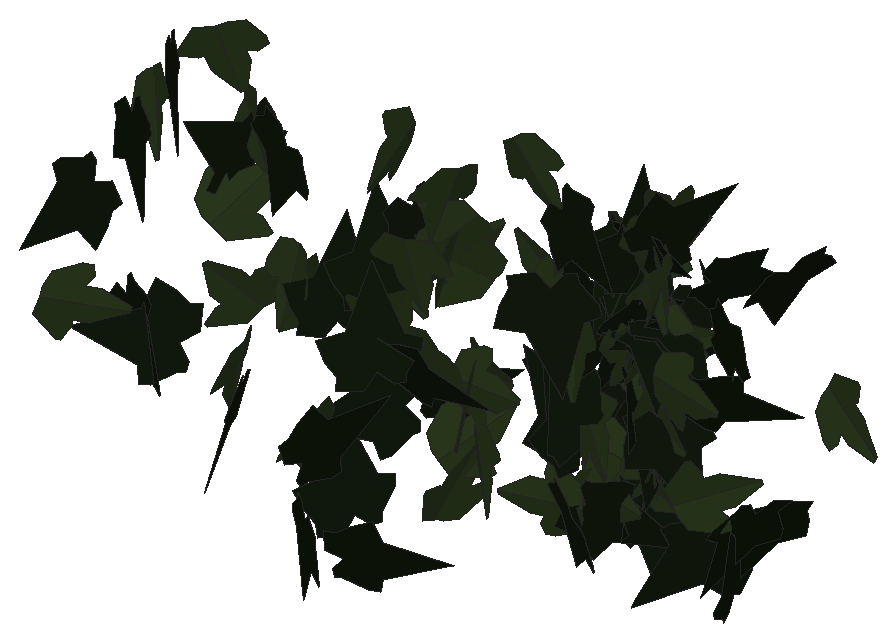
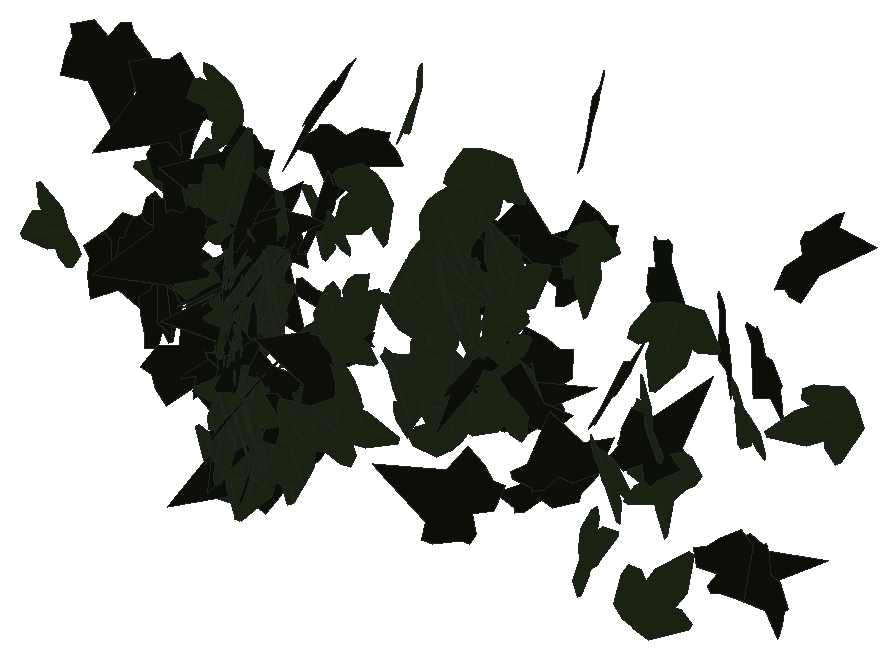
# SketchUp Ruby script. Lengths in inches.
U = 1.inch
M = Sketchup.active_model
def pt(a) = Geom::Point3d.new(a.map { |v| v * U })
def face(e, loops, mat)
  f = e.add_face(loops[0].map { |a| pt(a) })
  loops[1..].each { |l| e.add_face(l.map { |a| pt(a) }).erase! }
  f.material = f.back_material = mat if mat
  f
end
# faces: each face lists its corners as indices into pts; further lists are holes
def faces(e, pts, list, mat = nil) = list.each { |f| face(e, (f[0].is_a?(Array) ? f : [f]).map { |l| l.map { |i| pts[i] } }, mat) }
# xy, xz, yz: faces in a plane at the given z, y or x. An outline is a flat list of corners, or four numbers for a rectangle; further outlines are holes
def ring(l) = l.size == 4 ? [[l[0], l[1]], [l[2], l[1]], [l[2], l[3]], [l[0], l[3]]] : l.each_slice(2).to_a
def flat(e, list, mat, &to3) = list.each { |f| face(e, (f[0].is_a?(Array) ? f : [f]).map { |l| ring(l).map { |u, v| to3.(u, v) } }, mat) }
def xy(e, z, list, mat = nil) = flat(e, list, mat) { |x, y| [x, y, z] }
def xz(e, y, list, mat = nil) = flat(e, list, mat) { |x, z| [x, y, z] }
def yz(e, x, list, mat = nil) = flat(e, list, mat) { |y, z| [x, y, z] }
def lines(e, pts, list) = list.each { |a, b| e.add_line(pt(pts[a]), pt(pts[b])) }
# prism: a flat outline (further loops are holes) pulled along v
def prism(e, loops, v, mat = nil)
  f = face(e, loops, mat); d = Geom::Vector3d.new(v.map { |x| x * U })
  f.pushpull(f.normal.samedirection?(d) ? d.length : -d.length)
end
def box(e, o, s, mat = nil) = prism(e, [[o, [o[0] + s[0], o[1], o[2]], [o[0] + s[0], o[1] + s[1], o[2]], [o[0], o[1] + s[1], o[2]]]], [0, 0, s[2]], mat)
def at(x, y, z, deg = 0) = Geom::Transformation.translation(pt([x, y, z])) * Geom::Transformation.rotation(ORIGIN, Z_AXIS, deg.degrees)
def axes(o, x, y, z) = Geom::Transformation.new([*x, 0, *y, 0, *z, 0, *pt(o).to_a, 1])
def part(name) = M.definitions.add(name)
# library, detail: a bought-in or finely detailed component or shape, given as its bounding box
def library(name, o, s) = part(name).tap { |d| box(d.entities, o, s) }
def detail(e, o, s) = box(e.add_group.entities, o, s)
def put(e, d, t, mat = nil) = e.add_instance(d, t).tap { |i| i.material = mat if mat }
def group(e, t, mat = nil) = e.add_group.tap { |g| g.transformation = t; g.material = mat if mat }.entities
root = M.entities
M.materials.add("efeu1").color = [18, 25, 13]
M.materials.add("efeu2").color = [43, 57, 29]
c1 = part("ivyleaf_9")
p = [[1.54,2.16,1.25],[1.36,2.04,1.19],[-0.21,0.99,0.68],[-0.71,1.11,0.82],[-0.85,0.86,0.67],[-0.8,0.17,0.21],
  [-0.9,-0.01,0.1],[-0.67,-0.16,-0.02],[-0.08,-0.08,-0.05],[-0.03,-0.6,-0.4],[0.65,-0.88,-0.66],[0.83,-0.6,-0.49],
  [1.29,-0.42,-0.43],[1.8125,-0.07,-0.26],[1.21,0.44,0.15]]
faces(c1.entities,p,[[0,1,2,3,4,5,6,7,8,9,10,11,12,13,14]],"efeu1")
c2 = part("ivyleaf_10")
p = [[0,0.5,-0.03],[-0.0625,2.02,-0.43],[-0.19,2.01,-0.46],[-0.54,1.05,-0.29],[-0.52,0.625,-0.18],[-0.83,0.76,-0.28],
  [-1.16,0.64,-0.33],[-1.15,0.33,-0.24],[-0.77,-0.39,0.02],[-0.3,-0.51,0.16],[0.04,-0.48,0.23],[-0.02,2.01,-0.4375],
  [-0.06,2.01,-0.43],[0.04,-0.49,0.23],[0.67,-0.49,0.14],[1.38,0.36,-0.2],[1.375,0.51,-0.24],[0.81,0.65,-0.19],
  [0.62,0.59,-0.15],[0.6,1.09,-0.28],[0.5,1.23,-0.31]]
faces(c2.entities,p,[[0,1,2,3,4,5,6,7,8,9,10],[11,12,0,13,14,15,16,17,18,19,20]],"efeu2")
put(root,c1,axes([46.58,214.53,204.625],[0.12953,-0.08025,-0.47622],[0.43383,-0.19728,0.15125],[-0.21217,-0.45237,0.01852]))
put(root,c2,axes([48.01,216.6,205.49],[-0.16887,0.41664,-0.21885],[0.08584,-0.20134,-0.44955],[-0.46273,-0.1894,-0.00353]))
put(root,c1,axes([43.45,217.01,204.52],[-0.24461,0.1638,-0.40415],[0.33544,-0.22543,-0.29439],[-0.27866,-0.41515,0.00039]))
put(root,c2,axes([44.73,217.02,204.48],[-0.00248,-0.49033,-0.09783],[0.00039,0.09783,-0.49034],[0.49999,-0.00251,-0.00011]))
put(root,c1,axes([44.81,216.77,204.04],[0.04782,0.05091,0.4951],[0.37205,0.32672,-0.06954],[-0.3306,0.37505,-0.00664]))
put(root,c1,axes([40.19,217.84,206.26],[0.04779,-0.1253,-0.48168],[0.17581,-0.44845,0.1341],[-0.46562,-0.18219,0.0012]))
put(root,c1,axes([45.03,217.42,202.27],[0.27464,0.02878,0.41683],[0.41647,0.0212,-0.27587],[-0.03355,0.49872,-0.01233]))
put(root,c2,axes([39.43,218.0625,204.125],[-0.13123,-0.08103,-0.47562],[0.40132,0.25527,-0.15422],[0.26781,-0.42222,-0.00196]))
put(root,c1,axes([44.88,218.22,204.87],[-0.4693,-0.08253,0.15147],[0.15015,0.02067,0.47647],[-0.08491,0.49271,0.00538]))
put(root,c1,axes([44.95,218.68,204.66],[0.3334,-0.11638,0.35398],[0.33567,-0.11241,-0.35311],[0.16177,0.4731,0.00317]))
put(root,c2,axes([49.38,219.01,205.87],[-0.05167,0.02408,-0.49674],[0.45468,-0.20004,-0.05699],[-0.20148,-0.45761,-0.00123]))
put(root,c2,axes([44.91,218.91,206.4],[-0.49557,-0.06259,-0.02221],[0.02228,0.00085,-0.4995],[0.06257,-0.49607,0.00194]))
put(root,c2,axes([49.95,218.78,204.28],[-0.13303,-0.14946,0.45822],[0.2995,0.3468,0.20007],[-0.37763,0.32771,-0.00275]))
put(root,c1,axes([47.375,219.39,202.83],[0.0535,-0.26344,0.42159],[0.13056,-0.40169,-0.26757],[0.47968,0.13872,0.02581]))
put(root,c2,axes([44.28,219.19,204.8],[-0.43979,-0.11021,0.2108],[0.21019,0.02743,0.45285],[-0.11138,0.48693,0.0222]))
put(root,c1,axes([47.05,219.32,206.32],[-0.2296,-0.34172,-0.28375],[0.15592,0.23709,-0.41168],[0.4159,-0.27752,-0.00231]))
put(root,c1,axes([43.71,219.18,201.8],[-0.34448,-0.28067,0.22925],[0.18031,0.14162,0.44433],[-0.31435,0.3888,0.00364]))
put(root,c2,axes([45.11,219.26,204.65],[-0.42633,0.03899,0.2583],[-0.2573,0.02274,-0.42811],[-0.04514,-0.49796,0.00067]))
put(root,c2,axes([45.27,219.27,202.38],[-0.03263,-0.46023,0.19268],[0.02256,0.19154,0.46131],[-0.49842,0.0388,0.00826]))
put(root,c1,axes([44.12,219.71,203.34],[-0.24669,-0.16292,0.40324],[-0.33618,-0.22268,-0.29563],[0.27591,-0.41698,0.00033]))
put(root,c1,axes([50.45,219.52,203.9],[-0.10083,0.32672,-0.36481],[0.08409,-0.35538,-0.34152],[-0.48245,-0.13023,0.01672]))
put(root,c1,axes([49.99,219.68,202.51],[0.03718,0.28474,0.40932],[-0.12455,-0.39214,0.2841],[0.48281,-0.12309,0.04177]))
put(root,c2,axes([41.4,219.57,203.29],[0.11014,-0.48282,-0.06894],[-0.01346,0.06764,-0.49522],[0.48753,0.11095,0.0019]))
put(root,c2,axes([45.28,219.75,204.17],[0.30152,-0.33588,0.21511],[0.15163,-0.15288,-0.45126],[0.36891,0.33736,0.00966]))
put(root,c2,axes([45.3,219.73,204.15],[0.01351,-0.03269,-0.49875],[0.46164,-0.19043,0.02498],[-0.19158,-0.46116,0.02504]))
put(root,c2,axes([44.16,219.85,204.1],[-0.24019,-0.18747,0.39644],[-0.31777,-0.23709,-0.30465],[0.30221,-0.3983,-0.00526]))
put(root,c2,axes([45.25,219.45,203.2],[0.21624,0.14097,-0.42822],[0.33021,0.2738,0.25688],[0.30692,-0.3939,0.02532]))
put(root,c1,axes([50.47,219.89,203.73],[-0.05401,0.37275,-0.32885],[0.02679,-0.32812,-0.37632],[-0.49635,-0.05827,0.01547]))
put(root,c2,axes([46.94,219.96,205.47],[0.43784,-0.14719,0.1914],[0.18107,-0.06203,-0.46192],[0.15973,0.4738,-0.00102]))
put(root,c1,axes([46.95,219.76,207.34],[0.27159,-0.31176,-0.28115],[-0.17051,0.22408,-0.41318],[0.38362,0.32031,0.0154]))
put(root,c1,axes([39.13,220.05,205.98],[-0.19993,-0.00586,-0.45825],[0.45815,0.00959,-0.20001],[0.01114,-0.49987,0.00153]))
put(root,c1,axes([49.15,220.27,202.71],[0.00795,0.0842,-0.4928],[-0.0881,-0.48491,-0.08427],[-0.49211,0.08817,0.00712]))
put(root,c1,axes([47,219.97,203.97],[-0.43558,-0.07046,-0.23516],[-0.23223,-0.03705,0.44125],[-0.07961,0.49362,-0.00045]))
put(root,c1,axes([39.68,220.31,202.54],[-0.21443,-0.04391,0.44955],[-0.44194,-0.08245,-0.21885],[0.09335,-0.4912,-0.00346]))
put(root,c2,axes([46.6,220.23,202.4375],[0.00333,0.00641,0.49995],[-0.45133,-0.2151,0.00576],[0.21515,-0.45132,0.00436]))
put(root,c1,axes([38.78,220.4,202.85],[-0.09297,-0.02612,-0.49059],[0.48669,0.06321,-0.0956],[0.06701,-0.4953,0.01367]))
put(root,c1,axes([46.76,220.3,203.42],[-0.17843,-0.41597,0.21243],[0.08971,0.19265,0.45259],[-0.45838,0.19963,0.00588]))
put(root,c2,axes([44.4375,220.41,205.68],[0.20712,-0.45457,0.02166],[0.01295,-0.0179,-0.49951],[0.4549,0.20748,0.00436]))
put(root,c2,axes([44.4,220.51,206.63],[-0.08374,-0.47846,0.11859],[-0.02301,-0.11636,-0.48573],[0.4924,-0.08681,-0.00253]))
put(root,c2,axes([44.51,220.62,205.9375],[-0.20379,-0.25236,0.38051],[-0.23897,-0.29611,-0.32436],[0.38906,-0.31406,0.00008]))
put(root,c1,axes([46.77,220.3,205.45],[-0.07196,-0.31382,0.38254],[0.08253,0.37354,0.32196],[-0.48786,0.10948,-0.00196]))
put(root,c2,axes([44.6875,220.72,205.17],[-0.2269,-0.15427,-0.41799],[-0.34792,-0.23168,0.27437],[-0.27834,0.41536,-0.00221]))
put(root,c1,axes([46.96,220.3,202.5],[0.05035,0.05329,-0.4946],[0.24125,0.43213,0.07112],[0.43504,-0.24581,0.0178]))
put(root,c2,axes([46.77,220.68,202.61],[-0.03859,-0.02724,-0.49776],[0.43885,-0.23869,-0.02096],[-0.23648,-0.4385,0.04233]))
put(root,c2,axes([46.83,220.44,203.8],[-0.13247,0.47641,0.07408],[-0.03008,0.0685,-0.49437],[-0.48119,-0.13543,0.01051]))
put(root,c2,axes([44.8,220.74,203.46],[-0.26052,0.06545,0.42172],[0.40836,-0.10532,0.26861],[0.12399,0.48438,0.00142]))
put(root,c1,axes([39.22,220.81,206.67],[-0.12183,0.02353,-0.48436],[0.47615,-0.0888,-0.12408],[-0.09186,-0.49149,-0.00077]))
put(root,c1,axes([50.28,220.5,207.23],[-0.01143,0.48618,-0.11616],[0.00367,-0.11611,-0.48632],[-0.49986,-0.01197,-0.00091]))
put(root,c1,axes([49.24,220.57,205.46],[0.12817,-0.17916,0.44886],[-0.20597,0.39984,0.21841],[-0.4372,-0.24089,0.02869]))
put(root,c1,axes([49.05,220.43,206.72],[0.30306,0.27421,0.28804],[0.21668,0.18981,-0.40868],[-0.33347,0.37253,-0.00378]))
put(root,c1,axes([48.64,220.61,204.6],[0.36106,0.12356,0.32306],[0.30761,0.09881,-0.38159],[-0.15815,0.47431,-0.00467]))
put(root,c2,axes([41.21,220.97,204.04],[0.44389,-0.22854,0.02696],[0.02835,-0.00382,-0.49918],[0.22837,0.4447,0.00957]))
put(root,c2,axes([46.92,221.22,204.64],[-0.11615,0.21125,0.43804],[0.19888,-0.39035,0.24098],[0.44379,0.23022,0.00666]))
put(root,c2,axes([46.66,220.95,202.59],[-0.20869,-0.45093,-0.05577],[0.02323,0.0507,-0.49688],[0.45377,-0.20998,-0.00022]))
put(root,c2,axes([38.57,221.18,205.78],[0.36268,-0.15744,0.30606],[0.28263,-0.1175,-0.39537],[0.19642,0.45979,0.00376]))
put(root,c1,axes([46.92,221.35,203.84],[0.16273,-0.1436,-0.45044],[0.40843,-0.19724,0.21043],[-0.23813,-0.43643,0.0531]))
put(root,c1,axes([42.06,220.9,203.51],[-0.33382,-0.20922,0.30788],[0.25812,0.16786,0.39395],[-0.26821,0.42196,-0.00406]))
put(root,c2,axes([46.67,220.92,202.88],[0.07737,-0.01324,-0.4938],[0.48434,0.10028,0.0732],[0.09709,-0.48966,0.02834]))
put(root,c1,axes([47.21,221.1875,205.22],[-0.0687,0.30447,-0.39061],[0.08207,-0.3819,-0.31211],[-0.48841,-0.107,0.0025]))
put(root,c1,axes([42.83,220.92,204.24],[-0.48935,-0.03148,0.09772],[0.09758,0.00525,0.49036],[-0.03189,0.49898,0.00101]))
put(root,c1,axes([40.7,221.45,205.43],[0.02895,-0.36672,0.33864],[0.04442,-0.33597,-0.36763],[0.49718,0.05137,0.01313]))
put(root,c1,axes([47.55,221.2,203.59],[0.0642,-0.46248,-0.17885],[0.08086,0.1877,-0.45632],[0.48922,0.02967,0.09889]))
put(root,c2,axes([45.375,221.34,203.73],[-0.0051,0.01176,-0.49984],[0.40013,-0.29962,-0.01113],[-0.29979,-0.40011,-0.00635]))
put(root,c1,axes([47.15,221.45,205.03],[-0.02067,-0.49705,0.05018],[0.08858,-0.05307,-0.48922],[0.49166,-0.01133,0.09025]))
put(root,c1,axes([46.9,221.45,205.97],[-0.35075,-0.35634,-0.00043],[0.00038,0.00023,-0.5],[0.35634,-0.35075,0.00011]))
put(root,c1,axes([47.25,221.39,202.36],[-0.03016,-0.49312,-0.07697],[0.00802,0.07663,-0.49403],[0.49902,-0.03104,0.00329]))
put(root,c2,axes([45.08,221.24,206.99],[-0.40176,0.09441,-0.28227],[0.26644,-0.09725,-0.41176],[-0.13266,-0.48128,0.02783]))
put(root,c2,axes([47.05,221.32,203.67],[0.12877,-0.04202,0.4813],[0.48262,-0.01184,-0.13016],[0.02233,0.49809,0.03751]))
put(root,c2,axes([47.11,221.52,205.4],[0.10784,-0.39584,0.2858],[0.08719,-0.27236,-0.41014],[0.48038,0.1383,0.01028]))
put(root,c2,axes([46.94,221.38,202.48],[-0.02252,0.01152,0.49936],[0.4914,-0.08909,0.02422],[0.08954,0.49186,-0.00731]))
put(root,c1,axes([46.83,221.62,202.33],[0.15259,-0.15333,-0.45078],[0.37213,-0.25691,0.21335],[-0.29705,-0.40061,0.03571]))
put(root,c2,axes([45.6,220.89,204.95],[0.02539,-0.01982,-0.49896],[0.10338,0.48899,-0.01417],[0.48854,-0.10245,0.02893]))
put(root,c1,axes([45.8,220.98,203.92],[0.04989,0.00667,0.49746],[0.41707,0.272,-0.04548],[-0.27123,0.41949,0.02157]))
put(root,c2,axes([42.71,221.31,204.6],[0.36729,0.02431,0.33839],[0.33452,0.05715,-0.3672],[-0.05653,0.49613,0.02572]))
put(root,c2,axes([47.17,221.46,205.91],[0.32899,-0.12991,0.3534],[0.32928,-0.12831,-0.35371],[0.18259,0.46547,0.00113]))
put(root,c1,axes([46.83,221.35,205.14],[0.21219,-0.4288,-0.14528],[-0.06549,0.12969,-0.47843],[0.44798,0.22207,-0.00113]))
put(root,c2,axes([46.99,221.67,205.03],[-0.02738,0.03955,0.49768],[0.16842,-0.46848,0.0465],[0.46998,0.17019,0.01233]))
put(root,c2,axes([47.21,221.65,205.72],[0.05741,-0.1135,0.48355],[0.28365,-0.39209,-0.12571],[0.40773,0.28876,0.01937]))
put(root,c2,axes([46.98,221.46,202.74],[0.31031,-0.34934,-0.17797],[0.11784,-0.13337,0.46725],[-0.37393,-0.33193,-0.00044]))
put(root,c2,axes([47.16,221.52,202.88],[0.28351,-0.38538,0.14528],[0.08321,-0.11913,-0.47842],[0.40336,0.29545,-0.00341]))
put(root,c2,axes([46.71,221.4,205.41],[0.21224,-0.44942,-0.05451],[-0.02209,0.04985,-0.49702],[0.45218,0.21339,0.00131]))
put(root,c1,axes([43.38,221.24,202.6],[0.09631,-0.01856,0.49029],[0.49014,-0.01888,-0.09699],[0.02212,0.4993,0.01456]))
put(root,c2,axes([39.85,221.17,204.27],[0.32656,0.13338,-0.35435],[0.30499,0.18463,0.35056],[0.22437,-0.44511,0.03922]))
put(root,c2,axes([39.7,221.31,206.89],[-0.40499,-0.26957,-0.11539],[0.09602,0.06399,-0.4865],[0.27706,-0.41622,-0.00006]))
put(root,c1,axes([47,221.71,203.22],[0.02782,-0.45639,0.20231],[0.01076,-0.20203,-0.45724],[0.49911,0.0298,-0.00142]))
put(root,c2,axes([47.08,221.41,205.125],[0.46825,0.14372,0.10042],[0.09623,0.02872,-0.48981],[-0.14656,0.47804,-0.00076]))
put(root,c2,axes([47.21,221.6,204.73],[-0.3015,-0.14387,-0.37202],[-0.32897,-0.17402,0.33391],[-0.22555,0.44612,0.01027]))
put(root,c2,axes([42.48,221.79,206.1],[0.04934,-0.16108,0.47076],[0.18337,-0.43388,-0.16768],[0.46254,0.1892,0.01626]))
put(root,c1,axes([39.89,221.72,204.85],[0.06976,0.05189,0.49238],[-0.3815,-0.31131,0.08685],[0.31558,-0.38781,-0.00384]))
put(root,c2,axes([47.35,221.38,204.21],[0.05294,-0.47918,-0.13261],[0.0524,0.138,-0.47771],[0.49442,0.03669,0.06483]))
put(root,c2,axes([46.82,221.33,206.19],[-0.43729,0.16488,0.17774],[-0.16804,0.05811,-0.46732],[-0.17476,-0.46844,0.00459]))
put(root,c1,axes([46.98,221.32,205.76],[-0.2001,-0.28698,0.35721],[0.223,0.27952,0.34949],[-0.40029,0.29918,0.01613]))
put(root,c2,axes([47.19,221.73,206.35],[-0.0671,-0.39374,-0.30078],[-0.06263,-0.29435,0.39929],[-0.4915,0.09126,-0.00982]))
put(root,c2,axes([47.33,221.62,203.09],[0.28515,-0.38584,0.14079],[0.08323,-0.11356,-0.47977],[0.4022,0.29704,-0.00054]))
put(root,c2,axes([46.98,221.26,204.2],[-0.1072,-0.1456,0.46617],[0.30915,0.34924,0.18017],[-0.37807,0.32686,0.01515]))
put(root,c2,axes([46.97,221.58,202.32],[-0.11999,-0.48349,-0.04289],[0.00866,-0.0463,0.49778],[-0.48531,0.11871,0.01948]))
put(root,c2,axes([50.26,221.55,204.74],[0.22087,-0.0051,0.44854],[0.44856,-0.00153,-0.22089],[0.00362,0.49997,0.0039]))
put(root,c2,axes([47.1875,221.56,202.4375],[-0.0206,-0.49952,0.00754],[0.08748,-0.01103,-0.49217],[0.49186,-0.01896,0.08785]))
put(root,c2,axes([46.88,221.28,205.15],[0.137,-0.21893,-0.42814],[-0.23489,0.35798,-0.25822],[0.41959,0.27189,-0.00476]))
put(root,c1,axes([46.99,221.19,204.39],[0.22607,0.12204,0.42895],[0.38404,0.19121,-0.2568],[-0.22672,0.44558,-0.00728]))
put(root,c2,axes([46.85,221.44,202.39],[-0.4586,-0.17221,-0.10015],[0.09375,0.03524,-0.48987],[0.17577,-0.46809,-0.00003]))
put(root,c1,axes([46.96,221.35,206.23],[0.43915,0.12292,-0.20504],[-0.20006,-0.04583,-0.45594],[-0.13088,0.48248,0.00893]))
put(root,c2,axes([45.45,221.55,204.84],[-0.37014,0.03589,-0.33423],[-0.33225,0.03652,0.37186],[0.0511,0.49737,-0.00318]))
put(root,c1,axes([47.33,221.21,206.3125],[0.03758,0.04083,0.49691],[0.39183,0.30573,-0.05476],[-0.30831,0.39352,-0.00902]))
put(root,c1,axes([47.04,221.37,203.16],[0.46074,0.11666,-0.15527],[-0.15196,-0.03239,-0.47525],[-0.12094,0.48512,0.0056]))
put(root,c1,axes([42.93,221.5,205.21],[0.19836,-0.38174,-0.25481],[-0.09532,0.23727,-0.42967],[0.44896,0.21904,0.02136]))
put(root,c1,axes([47.15,221.7,205.1],[0.14021,-0.47986,0.00842],[0.18028,0.04453,-0.46424],[0.44479,0.13322,0.18551]))
put(root,c2,axes([47.09,221.47,204.67],[0.08651,-0.45029,-0.19939],[-0.03562,0.19619,-0.45852],[0.49117,0.09354,0.00187]))
put(root,c2,axes([40.81,221.91,203.14],[0.00236,0.13242,-0.48214],[-0.00805,-0.48207,-0.13244],[-0.49993,0.00839,-0.00015]))
put(root,c2,axes([47.09,221.52,201.85],[0.36859,-0.01292,-0.33761],[0.33727,-0.01517,0.3688],[-0.01977,-0.4996,-0.00247]))
put(root,c2,axes([43.86,221.1875,204.81],[0.03225,0.11375,-0.48582],[0.15505,0.46045,0.1181],[0.47426,-0.15827,-0.00557]))
put(root,c2,axes([47.11,221.56,203.56],[0.35142,-0.35313,0.04245],[-0.02883,0.0312,0.49819],[-0.3545,-0.3526,0.00157]))
put(root,c2,axes([39.82,221.85,202.56],[-0.27638,-0.22728,-0.34922],[-0.25652,-0.23741,0.35753],[-0.32834,0.3768,0.01463]))
put(root,c1,axes([46.96,221.45,203.5],[-0.45247,0.06984,0.20098],[0.19863,-0.03063,0.45783],[0.07627,0.49415,-0.00002]))
put(root,c1,axes([46.96,221.34,202.29],[0.01928,-0.01271,-0.49947],[0.12204,0.48482,-0.00762],[0.48449,-0.12162,0.0218]))
put(root,c1,axes([47.18,221.77,205.12],[0.05526,-0.48984,-0.08369],[0.11531,0.09455,-0.47725],[0.48337,0.03345,0.12342]))
put(root,c2,axes([46.83,221.88,204.71],[-0.05312,0.28242,-0.40917],[0.07265,-0.40267,-0.28736],[-0.49183,-0.08999,0.00175]))
put(root,c2,axes([47.05,221.42,206],[-0.14623,-0.25349,0.40541],[0.20111,0.35202,0.29264],[-0.43379,0.24865,-0.00099]))
put(root,c2,axes([39.71,221.82,205.46],[0.1518,-0.04412,0.47435],[0.44186,-0.17307,-0.1575],[0.17809,0.46701,-0.01355]))
put(root,c2,axes([47.04,221.38,204.97],[0.03587,-0.3019,-0.39695],[-0.03778,0.39519,-0.30397],[0.49728,0.05181,0.00554]))
put(root,c2,axes([47.09,221.46,204.55],[-0.1223,-0.10633,0.47301],[0.35716,0.31012,0.16206],[-0.32784,0.37752,0.0001]))
put(root,c2,axes([47.05,221.61,203.17],[-0.47774,-0.00599,0.1474],[-0.14718,-0.01487,-0.47762],[0.01011,-0.49974,0.01245]))
put(root,c2,axes([47.02,221.54,203.37],[0.28383,0.36901,0.18241],[0.10098,0.15238,-0.46539],[-0.39906,0.30102,0.01197]))
put(root,c2,axes([47.07,221.7,205.72],[0.14021,-0.47959,0.01822],[0.18053,0.03512,-0.46495],[0.44469,0.13696,0.183]))
put(root,c2,axes([46.91,221.52,204.62],[0.29632,0.38559,-0.11625],[0.07162,0.09158,0.4863],[0.39631,-0.30485,-0.00095]))
put(root,c1,axes([46.83,221.9375,204.03],[0.12508,-0.21495,0.43376],[0.21738,-0.37536,-0.24869],[0.43255,0.2508,-0.00045]))
